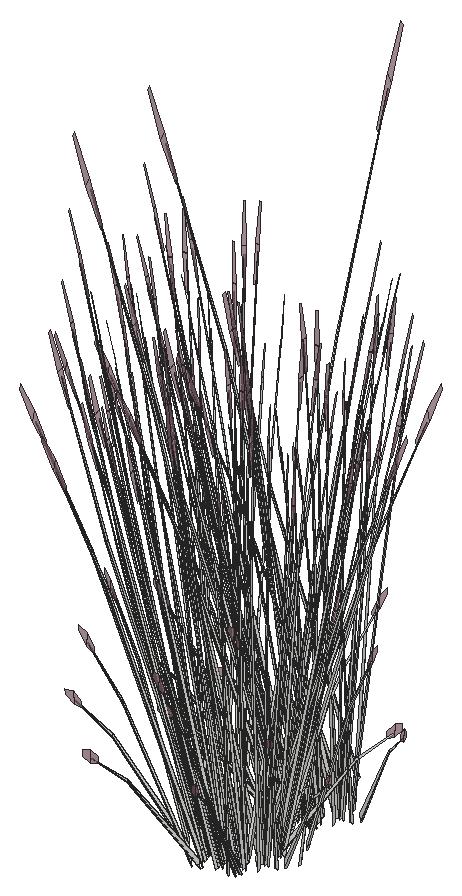
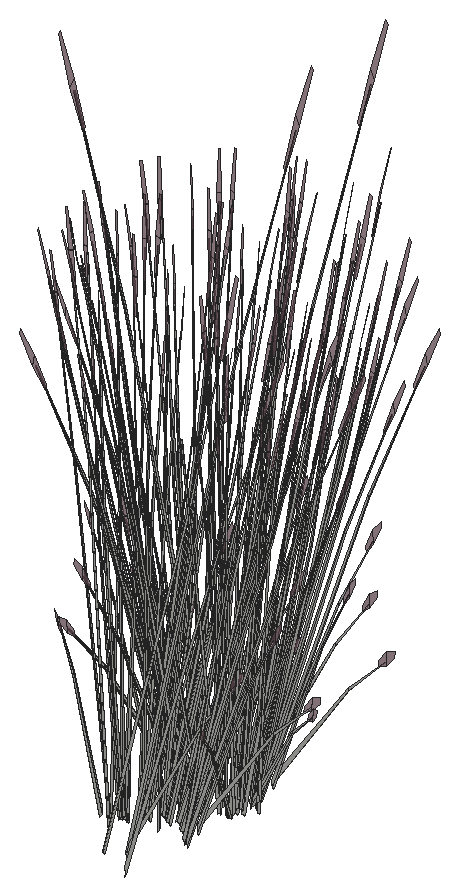
# SketchUp Ruby script. Lengths in inches.
U = 1.inch
M = Sketchup.active_model
def pt(a) = Geom::Point3d.new(a.map { |v| v * U })
def face(e, loops, mat)
  f = e.add_face(loops[0].map { |a| pt(a) })
  loops[1..].each { |l| e.add_face(l.map { |a| pt(a) }).erase! }
  f.material = f.back_material = mat if mat
  f
end
# faces: each face lists its corners as indices into pts; further lists are holes
def faces(e, pts, list, mat = nil) = list.each { |f| face(e, (f[0].is_a?(Array) ? f : [f]).map { |l| l.map { |i| pts[i] } }, mat) }
# xy, xz, yz: faces in a plane at the given z, y or x. An outline is a flat list of corners, or four numbers for a rectangle; further outlines are holes
def ring(l) = l.size == 4 ? [[l[0], l[1]], [l[2], l[1]], [l[2], l[3]], [l[0], l[3]]] : l.each_slice(2).to_a
def flat(e, list, mat, &to3) = list.each { |f| face(e, (f[0].is_a?(Array) ? f : [f]).map { |l| ring(l).map { |u, v| to3.(u, v) } }, mat) }
def xy(e, z, list, mat = nil) = flat(e, list, mat) { |x, y| [x, y, z] }
def xz(e, y, list, mat = nil) = flat(e, list, mat) { |x, z| [x, y, z] }
def yz(e, x, list, mat = nil) = flat(e, list, mat) { |y, z| [x, y, z] }
def lines(e, pts, list) = list.each { |a, b| e.add_line(pt(pts[a]), pt(pts[b])) }
# prism: a flat outline (further loops are holes) pulled along v
def prism(e, loops, v, mat = nil)
  f = face(e, loops, mat); d = Geom::Vector3d.new(v.map { |x| x * U })
  f.pushpull(f.normal.samedirection?(d) ? d.length : -d.length)
end
def box(e, o, s, mat = nil) = prism(e, [[o, [o[0] + s[0], o[1], o[2]], [o[0] + s[0], o[1] + s[1], o[2]], [o[0], o[1] + s[1], o[2]]]], [0, 0, s[2]], mat)
def at(x, y, z, deg = 0) = Geom::Transformation.translation(pt([x, y, z])) * Geom::Transformation.rotation(ORIGIN, Z_AXIS, deg.degrees)
def axes(o, x, y, z) = Geom::Transformation.new([*x, 0, *y, 0, *z, 0, *pt(o).to_a, 1])
def part(name) = M.definitions.add(name)
# library, detail: a bought-in or finely detailed component or shape, given as its bounding box
def library(name, o, s) = part(name).tap { |d| box(d.entities, o, s) }
def detail(e, o, s) = box(e.add_group.entities, o, s)
def put(e, d, t, mat = nil) = e.add_instance(d, t).tap { |i| i.material = mat if mat }
def group(e, t, mat = nil) = e.add_group.tap { |g| g.transformation = t; g.material = mat if mat }.entities
root = M.entities
M.materials.add("LightPink_Translucent").color = [144, 107, 117]
M.materials["LightPink_Translucent"].alpha = 0.75
c1 = part("blade")
p = [[2.15,0.21,22],[0,0.17,0],[0.09,0.45,0],[2.18,0.31,22],[2.29,0.31,22],[0.38,0.45,0],
  [2.48,0.24,33],[2.49,0.24,33],[2.48,0.22,33]]
faces(c1.entities,p,[[0,1,2,3],[4,5,2,3],[6,3,4,7],[8,0,3,6]])
c2 = part("seeds")
p = [[0.3,-0.1,1.38],[-0.01,-0.03,1.59],[-0.01,-0.03,0.03],[0.14,-0.07,-0.07],[0.29,-0.03,3],[0.15,0.01,3.11]]
faces(c2.entities,p,[[0,1,2,3],[1,0,4,5]],"LightPink_Translucent")
c3 = part("blade with seeds")
put(c3.entities,c1,at(0,0,0))
put(c3.entities,c2,axes([2.4,0.25,30.99],[1.5799,-0.05474,1.17369],[-0.12525,1.92788,0.29478],[-0.07173,-0.02425,1.56792]))
put(root,c3,axes([428.2,376.26,153.27],[0.09368,0.15143,1.44779],[-0.43286,0.12749,0.11706],[-0.09783,-0.23774,0.61892]))
put(root,c3,axes([428.91,375.26,153.98],[-0.06268,-0.06613,1.47793],[-0.4183,0.04193,-0.23373],[-0.06676,-0.15817,0.11853]))
put(root,c3,axes([429.35,376.375,154.21],[-0.19559,-0.38351,-0.60019],[0.40262,-0.21373,0.07243],[-0.04574,-0.1853,0.84903]))
put(root,c3,axes([430.17,376.75,154.21],[0.01066,-0.43628,-0.60019],[0.44902,0.0293,0.07243],[0.04739,-0.18483,0.84903]))
put(root,c3,axes([430.79,376.07,153.98],[-0.00396,-0.09387,1.47793],[-0.33411,-0.2713,-0.23373],[0.05166,-0.16446,0.11853]))
put(root,c3,axes([429.39,376.05,153.82],[0.12355,-0.36271,-0.29918],[0.36044,0.10579,0.38624],[-0.03305,-0.14603,0.73904]))
put(root,c3,axes([429.66,376.53,153.27],[-0.0763,0.16212,1.44779],[-0.3201,-0.3355,0.11706],[0.1444,-0.2091,0.61892]))
put(root,c3,axes([430.7,375.73,153.98],[-0.04162,0.03603,1.49853],[-0.40776,-0.12155,-0.1416],[-0.01476,-0.15722,0.26519]))
put(root,c3,axes([429.21,376.3,153.95],[-0.40284,-0.11824,-0.43168],[0.13808,-0.40538,-0.33437],[-0.03694,-0.16321,0.82598]))
put(root,c3,axes([430.08,376.6,153.95],[-0.29336,-0.31691,-0.43168],[0.3099,-0.27755,-0.33437],[0.04464,-0.16102,0.82598]))
put(root,c3,axes([428.49,375.04,153.98],[-0.00765,0.05653,1.49853],[-0.37706,0.20517,-0.1416],[-0.11096,-0.10488,0.26519]))
put(root,c3,axes([429.43,376.13,154],[0.4038,0.12331,0.40553],[-0.13808,0.40538,0.33437],[-0.02427,-0.15942,0.83914]))
put(root,c3,axes([429.55,376.28,154.25],[-0.40102,0.2196,-0.10273],[-0.19707,-0.38974,-0.57019],[-0.05291,-0.16424,0.8664]))
put(root,c3,axes([430.38,376.77,154.25],[-0.45039,-0.02337,-0.10273],[0.01231,-0.44247,-0.57019],[0.03129,-0.17041,0.8664]))
put(root,c3,axes([430.35,376.49,153.82],[0.27728,-0.24833,-0.29918],[0.26248,0.28355,0.38624],[0.03994,-0.14407,0.73904]))
put(root,c3,axes([429.54,376.1,154],[0.30197,-0.1603,0.05432],[0.1478,0.29231,0.42765],[-0.02916,-0.12885,0.65209]))
put(root,c3,axes([428.47,376.48,154.21],[-0.34944,-0.22798,-0.60019],[0.24834,-0.39949,0.07243],[-0.1266,-0.13612,0.84903]))
put(root,c3,axes([428.35,376.18,153.82],[-0.06329,-0.37991,-0.29918],[0.36182,-0.10032,0.38624],[-0.09718,-0.10887,0.73904]))
put(root,c3,axes([428.51,376.15,154],[0.18625,-0.29962,0.05432],[0.26523,0.17444,0.42765],[-0.08575,-0.09606,0.65209]))
put(root,c3,axes([427.57,376.73,153.27],[0.15222,0.08126,1.44779],[-0.31502,0.34091,0.11706],[-0.19634,-0.15379,0.61892]))
put(root,c3,axes([428.31,376.49,153.95],[-0.40438,0.11212,-0.43168],[-0.07074,-0.4246,-0.33437],[-0.10862,-0.12168,0.82598]))
put(root,c3,axes([430.35,376.58,154],[0.29182,0.32181,0.40553],[-0.3099,0.27755,0.33437],[0.05383,-0.15098,0.83914]))
put(root,c3,axes([428.59,376.12,154.59],[-0.2735,0.45217,-0.11506],[-0.39608,-0.2605,-0.63862],[-0.13768,-0.12775,0.97037]))
put(root,c3,axes([430.46,376.61,154],[0.33677,0.02198,0.05432],[-0.00923,0.33185,0.42765],[0.03524,-0.12712,0.65209]))
put(root,c3,axes([430.7,377.51,154.21],[0.21406,-0.37215,-0.60019],[0.37511,0.26448,0.07243],[0.12781,-0.13483,0.84903]))
put(root,c3,axes([430.6875,377.33,153.95],[-0.10528,-0.43067,-0.43168],[0.39868,-0.07534,-0.33437],[0.11425,-0.11568,0.82598]))
put(root,c3,axes([427.54,375.99,153.98],[-0.08817,-0.00333,1.47793],[-0.28072,0.33293,-0.23373],[-0.14978,-0.06803,0.11853]))
put(root,c3,axes([430.875,377.64,154.25],[-0.37908,-0.26007,-0.10273],[0.21839,-0.37663,-0.57019],[0.1071,-0.13092,0.8664]))
put(root,c3,axes([429.31,379.0625,152.81],[0.35414,0.19019,1.27785],[-0.34693,0.40974,0.50532],[-0.1554,-0.24285,1.07126]))
put(root,c3,axes([431.81,377.53,153.98],[-0.05353,-0.00358,1.49853],[-0.22227,-0.38383,-0.1416],[0.08926,-0.1262,0.26519]))
put(root,c3,axes([430.98,377.38,153.82],[0.35672,-0.06741,-0.29918],[0.09419,0.38534,0.38624],[0.10222,-0.1035,0.73904]))
put(root,c3,axes([427.63,376.74,154],[0.02064,-0.35866,0.05432],[0.3116,0.00983,0.42765],[-0.11936,-0.03753,0.65209]))
put(root,c3,axes([427.51,376.85,153.82],[-0.23317,-0.29531,-0.29918],[0.26625,-0.27955,0.38624],[-0.13527,-0.04253,0.73904]))
put(root,c3,axes([427.76,377.05,154.21],[-0.40965,-0.01136,-0.60019],[0.02751,-0.47821,0.07243],[-0.17355,-0.05047,0.84903]))
put(root,c3,axes([431.01,377.55,154],[0.28133,0.19836,0.05432],[-0.16379,0.28248,0.42765],[0.0902,-0.09132,0.65209]))
put(root,c3,axes([430.93,377.46,154],[0.10163,0.43409,0.40553],[-0.39868,0.07534,0.33437],[0.1175,-0.10209,0.83914]))
put(root,c3,axes([432.01,377.99,153.98],[0.05687,-0.07184,1.47793],[-0.07279,-0.44069,-0.23373],[0.14268,-0.08356,0.11853]))
put(root,c3,axes([427.2,376.27,153.98],[0.03038,0.04707,1.49853],[-0.14646,0.42312,-0.1416],[-0.14833,0.00306,0.26519]))
put(root,c3,axes([427.625,377.14,153.95],[-0.29757,0.31243,-0.43168],[-0.2606,-0.33005,-0.33437],[-0.15119,-0.04754,0.82598]))
put(root,c3,axes([427.78,376.82,154.25],[-0.02194,0.47967,-0.10273],[-0.41546,-0.01311,-0.57019],[-0.16001,-0.03332,0.8664]))
put(root,c3,axes([430.89,378.66,154.25],[-0.20619,-0.42709,-0.10273],[0.36595,-0.20988,-0.57019],[0.15422,-0.05635,0.8664]))
put(root,c3,axes([430.87,378.29,153.95],[0.11102,-0.42903,-0.43168],[0.38064,0.14706,-0.33437],[0.15325,-0.03934,0.82598]))
put(root,c3,axes([427.25,377.48,153.27],[0.16998,-0.01068,1.44779],[-0.11276,0.46299,0.11706],[-0.24224,-0.02864,0.61892]))
put(root,c3,axes([430.8,378.45,154.21],[0.3601,-0.20831,-0.60019],[0.20068,0.4288,0.07243],[0.17399,-0.04871,0.84903]))
put(root,c3,axes([427.18,377.83,154],[0.11578,-0.43006,0.40553],[0.38064,0.14706,0.33437],[-0.14969,0.02584,0.83914]))
put(root,c3,axes([427.15,377.71,154],[-0.15051,-0.3216,0.05432],[0.27447,-0.15741,0.42765],[-0.12099,0.03106,0.65209]))
put(root,c3,axes([428.2,382.01,153.27],[0.09368,0.15143,1.44779],[-0.43286,0.12749,0.11706],[-0.09783,-0.23774,0.61892]))
put(root,c3,axes([428.91,381.01,153.98],[-0.06268,-0.06613,1.47793],[-0.4183,0.04193,-0.23373],[-0.06676,-0.15817,0.11853]))
put(root,c3,axes([431.1,378.49,153.82],[0.34057,0.13158,-0.29918],[-0.09933,0.38387,0.38624],[0.13712,-0.0352,0.73904]))
put(root,c3,axes([429.35,382.12,154.21],[-0.19559,-0.38351,-0.60019],[0.40262,-0.21373,0.07243],[-0.04574,-0.1853,0.84903]))
put(root,c3,axes([427.1,377.875,153.82],[-0.34057,-0.13158,-0.29918],[0.09933,-0.38387,0.38624],[-0.13712,0.0352,0.73904]))
put(root,c3,axes([430.18,378.01,153.27],[-0.16998,0.01068,1.44779],[0.11276,-0.46299,0.11706],[0.24224,0.02864,0.61892]))
put(root,c3,axes([430.17,382.5,154.21],[0.01066,-0.43628,-0.60019],[0.44902,0.0293,0.07243],[0.04739,-0.18483,0.84903]))
put(root,c3,axes([431.05,378.65,154],[0.15051,0.3216,0.05432],[-0.27447,0.15741,0.42765],[0.12099,-0.03106,0.65209]))
put(root,c3,axes([430.79,381.82,153.98],[-0.00396,-0.09387,1.47793],[-0.33411,-0.2713,-0.23373],[0.05166,-0.16446,0.11853]))
put(root,c3,axes([429.39,381.8,153.82],[0.12355,-0.36271,-0.29918],[0.36044,0.10579,0.38624],[-0.03305,-0.14603,0.73904]))
put(root,c3,axes([429.66,382.28,153.27],[-0.0763,0.16212,1.44779],[-0.3201,-0.3355,0.11706],[0.1444,-0.2091,0.61892]))
put(root,c3,axes([431.03,378.53,154],[-0.11578,0.43006,0.40553],[-0.38064,-0.14706,0.33437],[0.14969,-0.02584,0.83914]))
put(root,c3,axes([430.7,381.48,153.98],[-0.04162,0.03603,1.49853],[-0.40776,-0.12155,-0.1416],[-0.01476,-0.15722,0.26519]))
put(root,c3,axes([429.21,382.05,153.95],[-0.40284,-0.11824,-0.43168],[0.13808,-0.40538,-0.33437],[-0.03694,-0.16321,0.82598]))
put(root,c3,axes([430.08,382.35,153.95],[-0.29336,-0.31691,-0.43168],[0.3099,-0.27755,-0.33437],[0.04464,-0.16102,0.82598]))
put(root,c3,axes([428.14,377.8125,152.82],[0.11649,-0.06823,1.49584],[0.04017,0.47639,0.11706],[-0.25231,0.06321,0.53462]))
put(root,c3,axes([428.49,380.79,153.98],[-0.00765,0.05653,1.49853],[-0.37706,0.20517,-0.1416],[-0.11096,-0.10488,0.26519]))
put(root,c3,axes([429.43,381.88,154],[0.4038,0.12331,0.40553],[-0.13808,0.40538,0.33437],[-0.02427,-0.15942,0.83914]))
put(root,c3,axes([431.71,379.93,153.98],[-0.03706,-0.04129,1.49853],[0.08106,-0.44261,-0.1416],[0.14596,-0.02828,0.26519]))
put(root,c3,axes([429.55,382.03,154.25],[-0.40102,0.2196,-0.10273],[-0.19707,-0.38974,-0.57019],[-0.05291,-0.16424,0.8664]))
put(root,c3,axes([430.38,382.52,154.25],[-0.45039,-0.02337,-0.10273],[0.01231,-0.44247,-0.57019],[0.03129,-0.17041,0.8664]))
put(root,c3,axes([430.35,382.23,153.82],[0.27728,-0.24833,-0.29918],[0.26248,0.28355,0.38624],[0.03994,-0.14407,0.73904]))
put(root,c3,axes([429.54,381.85,154],[0.30197,-0.1603,0.05432],[0.1478,0.29231,0.42765],[-0.02916,-0.12885,0.65209]))
put(root,c3,axes([428.47,382.23,154.21],[-0.34944,-0.22798,-0.60019],[0.24834,-0.39949,0.07243],[-0.1266,-0.13612,0.84903]))
put(root,c3,axes([426.89,378.13,153.98],[-0.06692,0.06124,1.47793],[0.00569,0.44742,-0.23373],[-0.15339,0.05818,0.11853]))
put(root,c3,axes([427.34,378.07,153.95],[-0.11102,0.42903,-0.43168],[-0.38064,-0.14706,-0.33437],[-0.15325,0.03934,0.82598]))
put(root,c3,axes([427.32,377.7,154.25],[0.20619,0.42709,-0.10273],[-0.36595,0.20988,-0.57019],[-0.15422,0.05635,0.8664]))
put(root,c3,axes([428.35,381.93,153.82],[-0.06329,-0.37991,-0.29918],[0.36182,-0.10032,0.38624],[-0.09718,-0.10887,0.73904]))
put(root,c3,axes([431.39,379.56,153.32],[-0.07843,-0.39649,-0.0295],[0.37072,-0.09115,-0.13375],[0.07742,0.02514,0.44114]))
put(root,c3,axes([430.43,379.54,154.25],[0.02194,-0.47967,-0.10273],[0.41546,0.01311,-0.57019],[0.16001,0.03332,0.8664]))
put(root,c3,axes([428.51,381.89,154],[0.18625,-0.29962,0.05432],[0.26523,0.17444,0.42765],[-0.08575,-0.09606,0.65209]))
put(root,c3,axes([427.57,382.48,153.27],[0.15222,0.08126,1.44779],[-0.31502,0.34091,0.11706],[-0.19634,-0.15379,0.61892]))
put(root,c3,axes([430.79,379.26,153.98],[0.08791,-0.00798,1.47793],[0.24113,-0.36643,-0.23373],[0.15637,0.04837,0.11853]))
put(root,c3,axes([427.27,378.9,154],[-0.10163,-0.43409,0.40553],[0.39868,-0.07534,0.33437],[-0.1175,0.10209,0.83914]))
put(root,c3,axes([428.31,382.24,153.95],[-0.40438,0.11212,-0.43168],[-0.07074,-0.4246,-0.33437],[-0.10862,-0.12168,0.82598]))
put(root,c3,axes([430.35,382.33,154],[0.29182,0.32181,0.40553],[-0.3099,0.27755,0.33437],[0.05383,-0.15098,0.83914]))
put(root,c3,axes([427.19,378.81,154],[-0.28133,-0.19836,0.05432],[0.16379,-0.28248,0.42765],[-0.0902,0.09132,0.65209]))
put(root,c3,axes([427.32,378.29,153.27],[0.14219,-0.09977,1.44779],[0.11971,0.461,0.11706],[-0.22323,0.10419,0.61892]))
put(root,c3,axes([428.59,381.86,154.59],[-0.2735,0.45217,-0.11506],[-0.39608,-0.2605,-0.63862],[-0.13768,-0.12775,0.97037]))
put(root,c3,axes([430.46,382.36,154],[0.33677,0.02198,0.05432],[-0.00923,0.33185,0.42765],[0.03524,-0.12712,0.65209]))
put(root,c3,axes([430.7,383.26,154.21],[0.21406,-0.37215,-0.60019],[0.37511,0.26448,0.07243],[0.12781,-0.13483,0.84903]))
put(root,c3,axes([430.45,379.3125,154.21],[0.40965,0.01136,-0.60019],[-0.02751,0.47821,0.07243],[0.17355,0.05047,0.84903]))
put(root,c3,axes([430.6875,383.08,153.95],[-0.10528,-0.43067,-0.43168],[0.39868,-0.07534,-0.33437],[0.11425,-0.11568,0.82598]))
put(root,c3,axes([427.54,381.73,153.98],[-0.08817,-0.00333,1.47793],[-0.28072,0.33293,-0.23373],[-0.14978,-0.06803,0.11853]))
put(root,c3,axes([430.875,383.39,154.25],[-0.37908,-0.26007,-0.10273],[0.21839,-0.37663,-0.57019],[0.1071,-0.13092,0.8664]))
put(root,c3,axes([426.14,378.58,153.98],[0.0523,0.01265,1.49853],[0.16179,0.41674,-0.1416],[-0.10706,0.10938,0.26519]))
put(root,c3,axes([430.69,379.51,153.82],[0.23317,0.29531,-0.29918],[-0.26625,0.27955,0.38624],[0.13527,0.04253,0.73904]))
put(root,c3,axes([429.31,384.81,152.81],[0.35414,0.19019,1.27785],[-0.34693,0.40974,0.50532],[-0.1554,-0.24285,1.07126]))
put(root,c3,axes([430.57,379.625,154],[-0.02064,0.35866,0.05432],[-0.3116,-0.00983,0.42765],[0.11936,0.03753,0.65209]))
put(root,c3,axes([427.23,378.98,153.82],[-0.35672,0.06741,-0.29918],[-0.09419,-0.38534,0.38624],[-0.10222,0.1035,0.73904]))
put(root,c3,axes([431.81,383.28,153.98],[-0.05353,-0.00358,1.49853],[-0.22227,-0.38383,-0.1416],[0.08926,-0.1262,0.26519]))
put(root,c3,axes([430.6,379.51,154],[-0.30217,0.31079,0.40553],[-0.2606,-0.33005,0.33437],[0.14177,0.05733,0.83914]))
put(root,c3,axes([430.98,383.13,153.82],[0.35672,-0.06741,-0.29918],[0.09419,0.38534,0.38624],[0.10222,-0.1035,0.73904]))
put(root,c3,axes([427.63,382.48,154],[0.02064,-0.35866,0.05432],[0.3116,0.00983,0.42765],[-0.11936,-0.03753,0.65209]))
put(root,c3,axes([427.51,382.6,153.82],[-0.23317,-0.29531,-0.29918],[0.26625,-0.27955,0.38624],[-0.13527,-0.04253,0.73904]))
put(root,c3,axes([429.86,378.75,153.27],[-0.15222,-0.08126,1.44779],[0.31502,-0.34091,0.11706],[0.19634,0.15379,0.61892]))
put(root,c3,axes([429.88,377.68,153.78],[-0.35411,-0.24507,1.16821],[0.37391,-0.38156,0.50405],[0.11425,0.22994,1.12919]))
put(root,c3,axes([427.33,378.72,154.25],[0.37908,0.26007,-0.10273],[-0.21839,0.37663,-0.57019],[-0.1071,0.13092,0.8664]))
put(root,c3,axes([429.61,380.07,154.25],[0.2442,-0.40372,-0.10273],[0.35364,0.23259,-0.57019],[0.12293,0.11406,0.8664]))
put(root,c3,axes([427.84,378.6,153.27],[0.10236,-0.14492,1.44779],[0.25844,0.39118,0.11706],[-0.17726,0.17814,0.61892]))
put(root,c3,axes([427.52,379.03,153.95],[0.10528,0.43067,-0.43168],[-0.39868,0.07534,-0.33437],[-0.11425,0.11568,0.82598]))
put(root,c3,axes([427.76,382.79,154.21],[-0.40965,-0.01136,-0.60019],[0.02751,-0.47821,0.07243],[-0.17355,-0.05047,0.84903]))
put(root,c3,axes([429.29,380.4,153.98],[0.00121,-0.0571,1.49853],[0.35119,-0.25193,-0.1416],[0.12199,0.08992,0.26519]))
put(root,c3,axes([427.75,379.75,154],[-0.33677,-0.02198,0.05432],[0.00923,-0.33185,0.42765],[-0.03524,0.12712,0.65209]))
put(root,c3,axes([431.01,383.29,154],[0.28133,0.19836,0.05432],[-0.16379,0.28248,0.42765],[0.0902,-0.09132,0.65209]))
put(root,c3,axes([427.85,379.78,154],[-0.29182,-0.32181,0.40553],[0.3099,-0.27755,0.33437],[-0.05383,0.15098,0.83914]))
put(root,c3,axes([429.9,379.87,153.95],[0.40438,-0.11212,-0.43168],[0.07074,0.4246,-0.33437],[0.10862,0.12168,0.82598]))
put(root,c3,axes([430.93,383.21,154],[0.10163,0.43409,0.40553],[-0.39868,0.07534,0.33437],[0.1175,-0.10209,0.83914]))
put(root,c3,axes([432.01,383.74,153.98],[0.05687,-0.07184,1.47793],[-0.07279,-0.44069,-0.23373],[0.14268,-0.08356,0.11853]))
put(root,c3,axes([427.2,382.02,153.98],[0.03038,0.04707,1.49853],[-0.14646,0.42312,-0.1416],[-0.14833,0.00306,0.26519]))
put(root,c3,axes([429.7,380.21,154],[-0.18625,0.29962,0.05432],[-0.26523,-0.17444,0.42765],[0.08575,0.09606,0.65209]))
put(root,c3,axes([427.625,382.89,153.95],[-0.29757,0.31243,-0.43168],[-0.2606,-0.33005,-0.33437],[-0.15119,-0.04754,0.82598]))
put(root,c3,axes([429.78,380.13,154],[-0.4076,0.10824,0.40553],[-0.07074,-0.4246,0.33437],[0.09586,0.12514,0.83914]))
put(root,c3,axes([428.2,386.58,153.27],[0.09368,0.15143,1.44779],[-0.43286,0.12749,0.11706],[-0.09783,-0.23774,0.61892]))
put(root,c3,axes([427.77,378.96,153.27],[0.0763,-0.16212,1.44779],[0.3201,0.3355,0.11706],[-0.1444,0.2091,0.61892]))
put(root,c3,axes([428.91,385.58,153.98],[-0.06268,-0.06613,1.47793],[-0.4183,0.04193,-0.23373],[-0.06676,-0.15817,0.11853]))
put(root,c3,axes([427.78,382.5625,154.25],[-0.02194,0.47967,-0.10273],[-0.41546,-0.01311,-0.57019],[-0.16001,-0.03332,0.8664]))
put(root,c3,axes([430.89,384.41,154.25],[-0.20619,-0.42709,-0.10273],[0.36595,-0.20988,-0.57019],[0.15422,-0.05635,0.8664]))
put(root,c3,axes([430.87,384.04,153.95],[0.11102,-0.42903,-0.43168],[0.38064,0.14706,-0.33437],[0.15325,-0.03934,0.82598]))
put(root,c3,axes([429.35,386.69,154.21],[-0.19559,-0.38351,-0.60019],[0.40262,-0.21373,0.07243],[-0.04574,-0.1853,0.84903]))
put(root,c3,axes([428.66,380.26,154],[-0.30197,0.1603,0.05432],[-0.1478,-0.29231,0.42765],[0.02916,0.12885,0.65209]))
put(root,c3,axes([427.85,379.875,153.82],[-0.27728,0.24833,-0.29918],[-0.26248,-0.28355,0.38624],[-0.03994,0.14407,0.73904]))
put(root,c3,axes([426.9,379.8,153.98],[-0.01019,0.09334,1.47793],[0.28908,0.3247,-0.23373],[-0.07568,0.15355,0.11853]))
